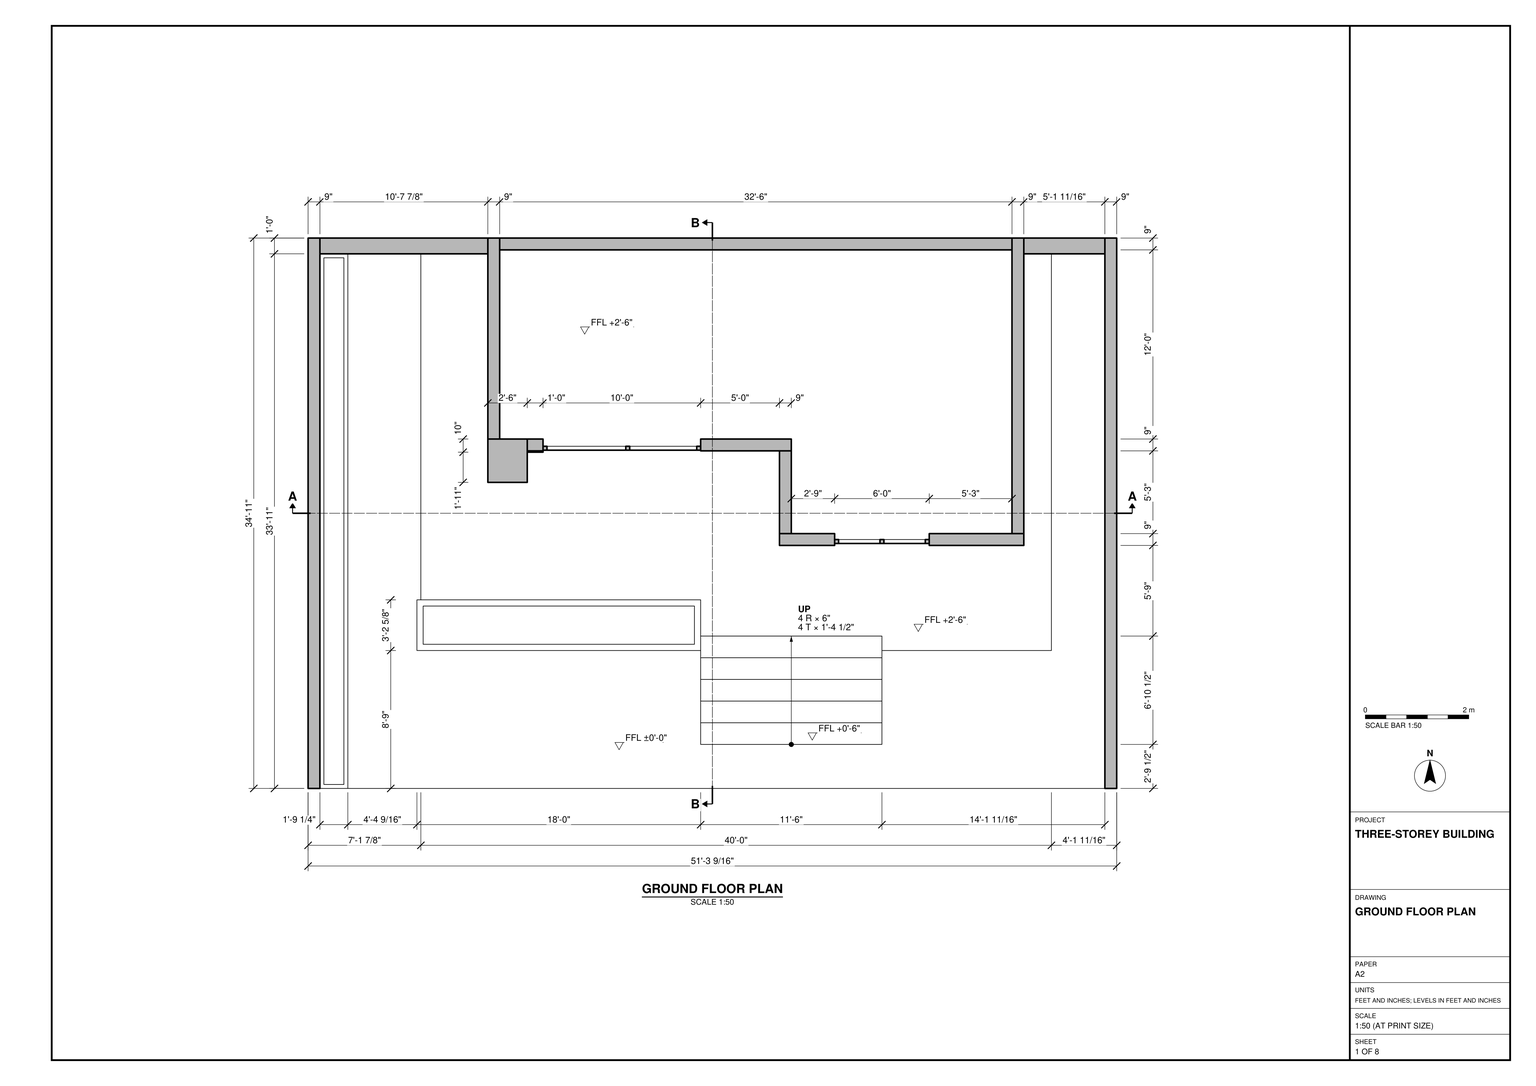
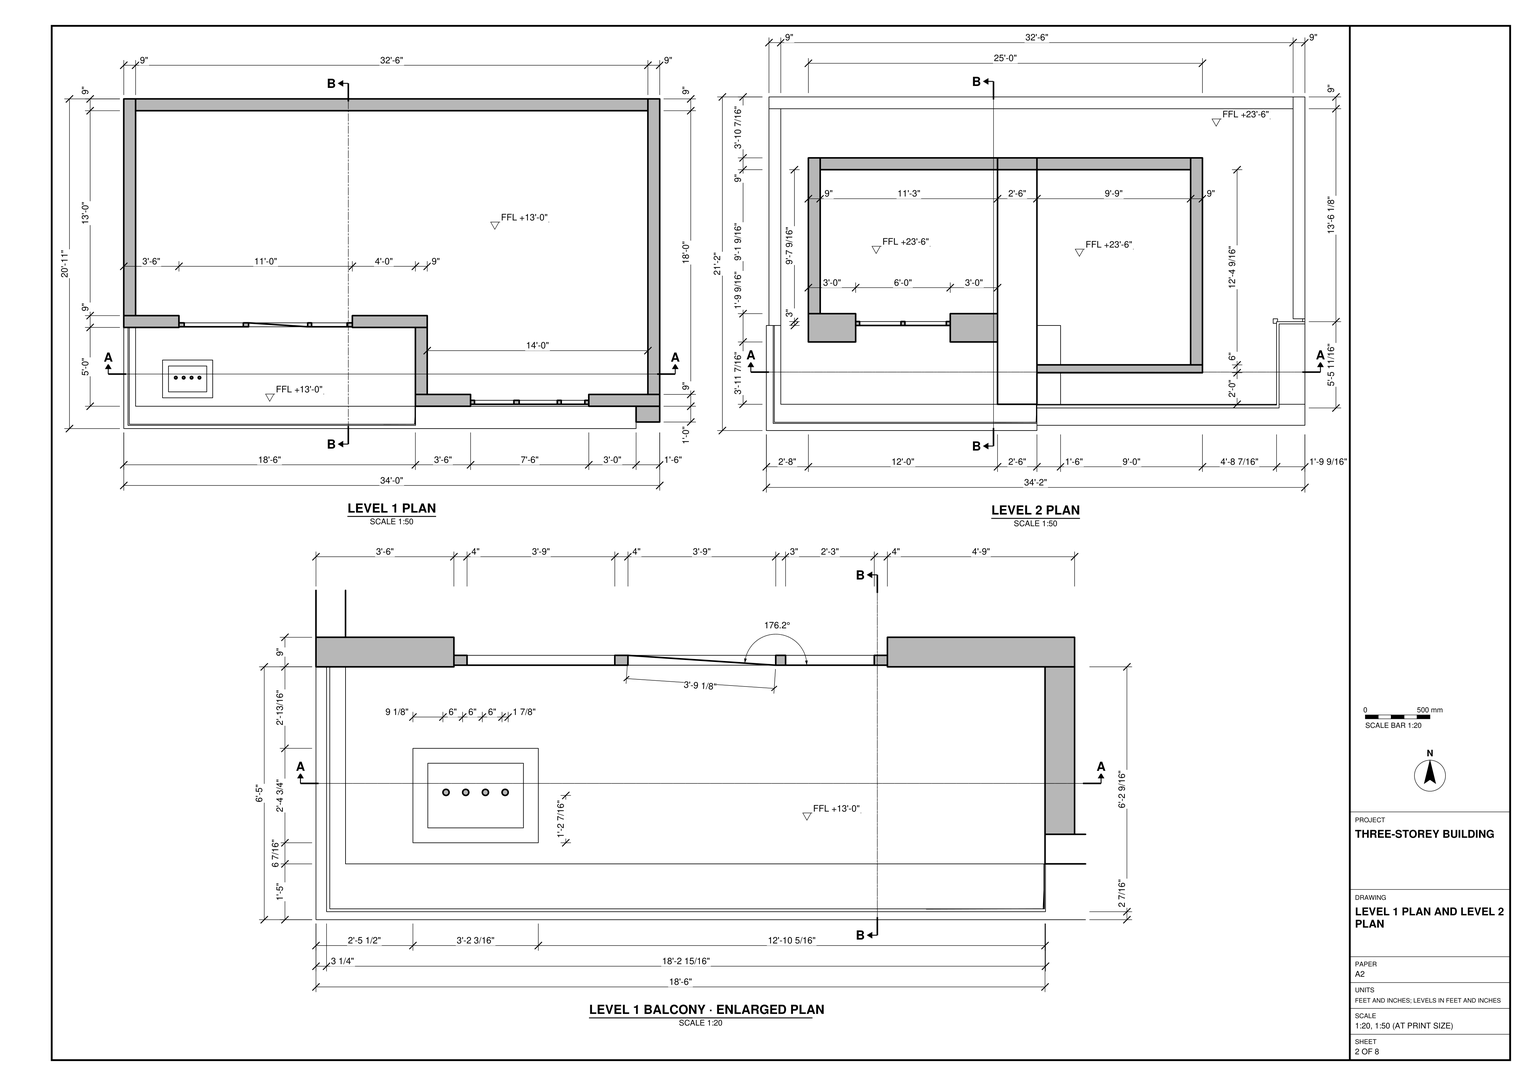
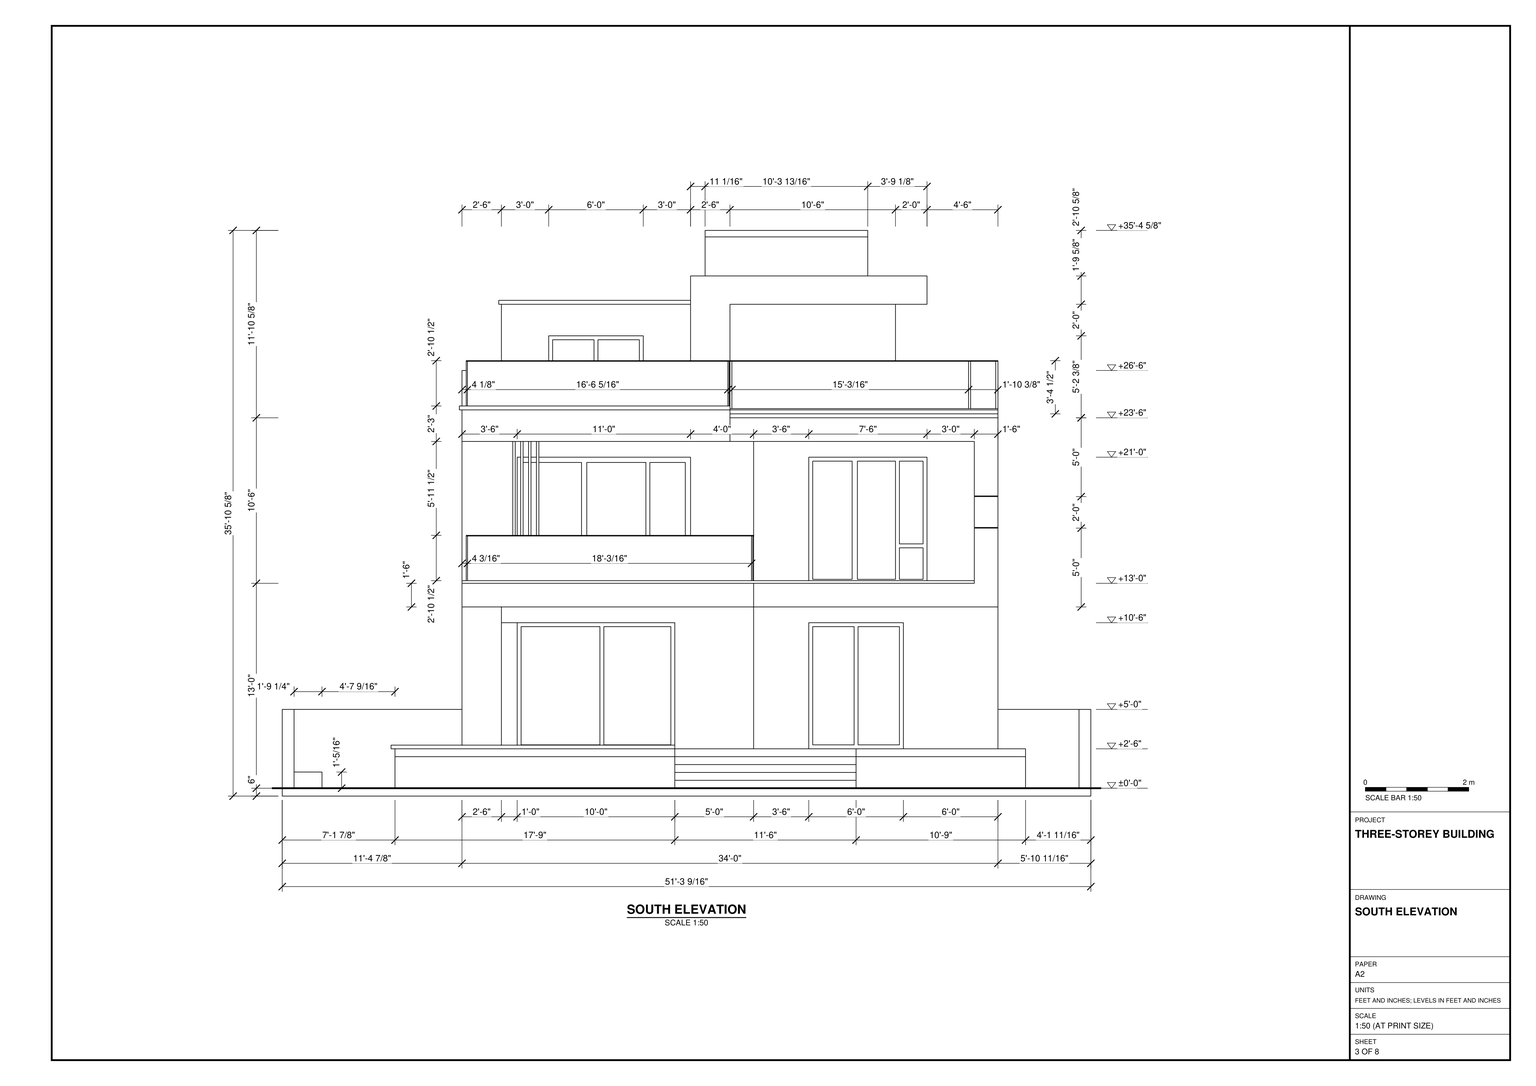
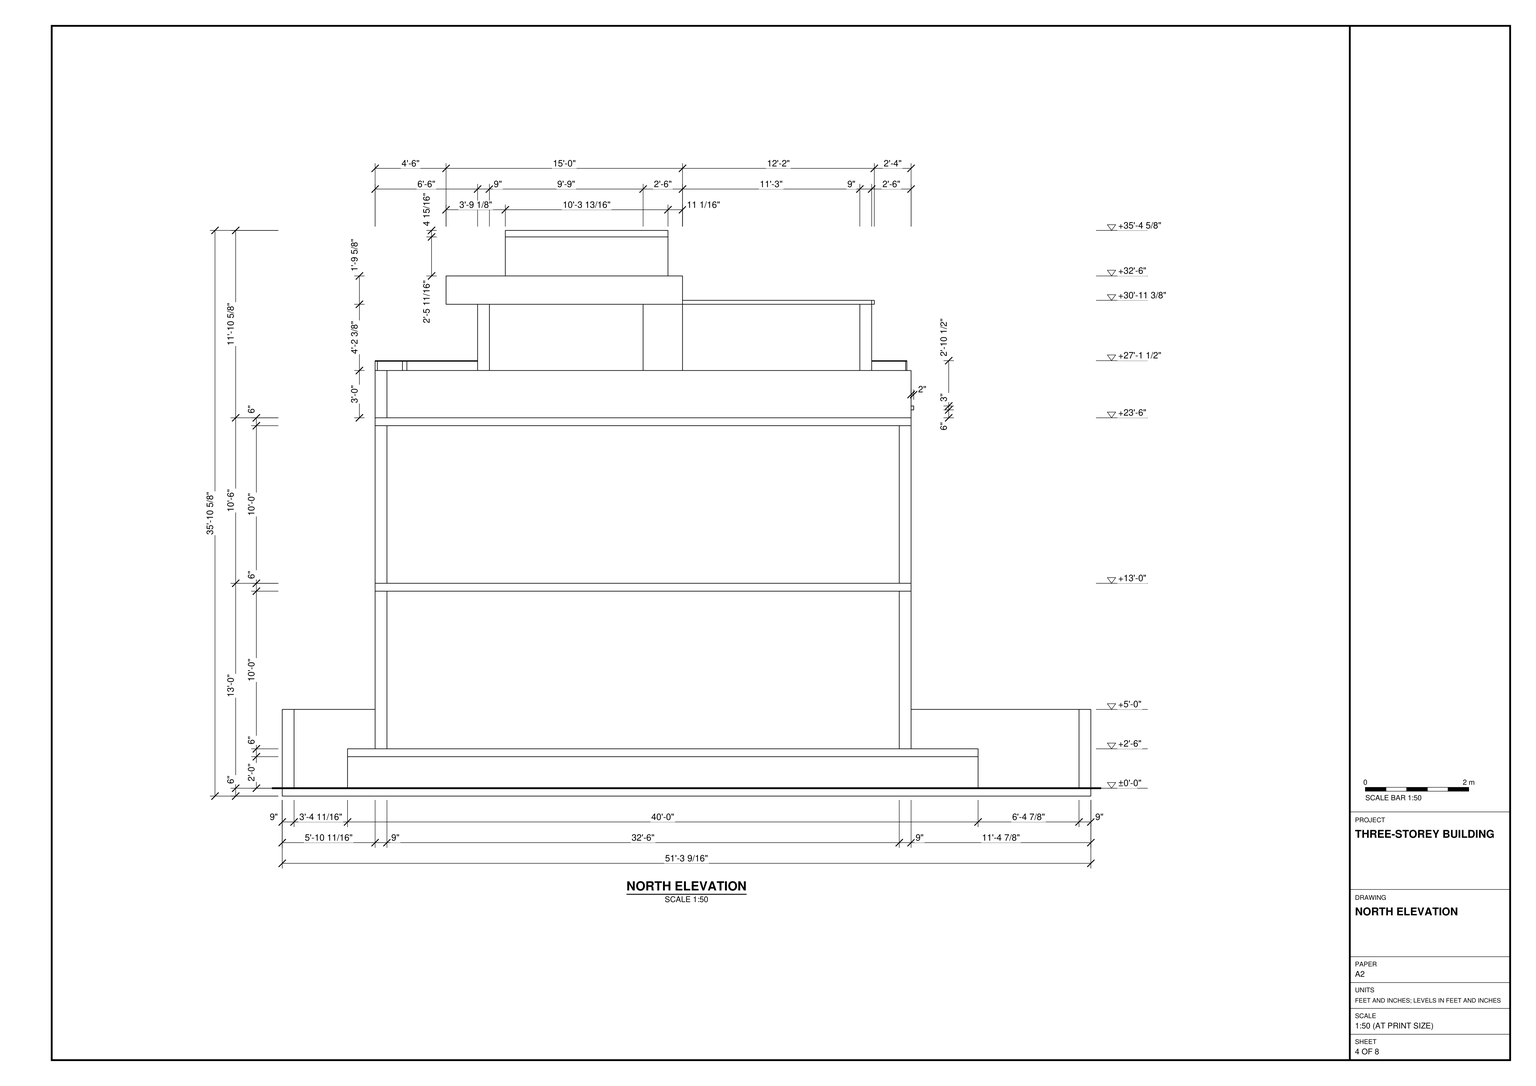
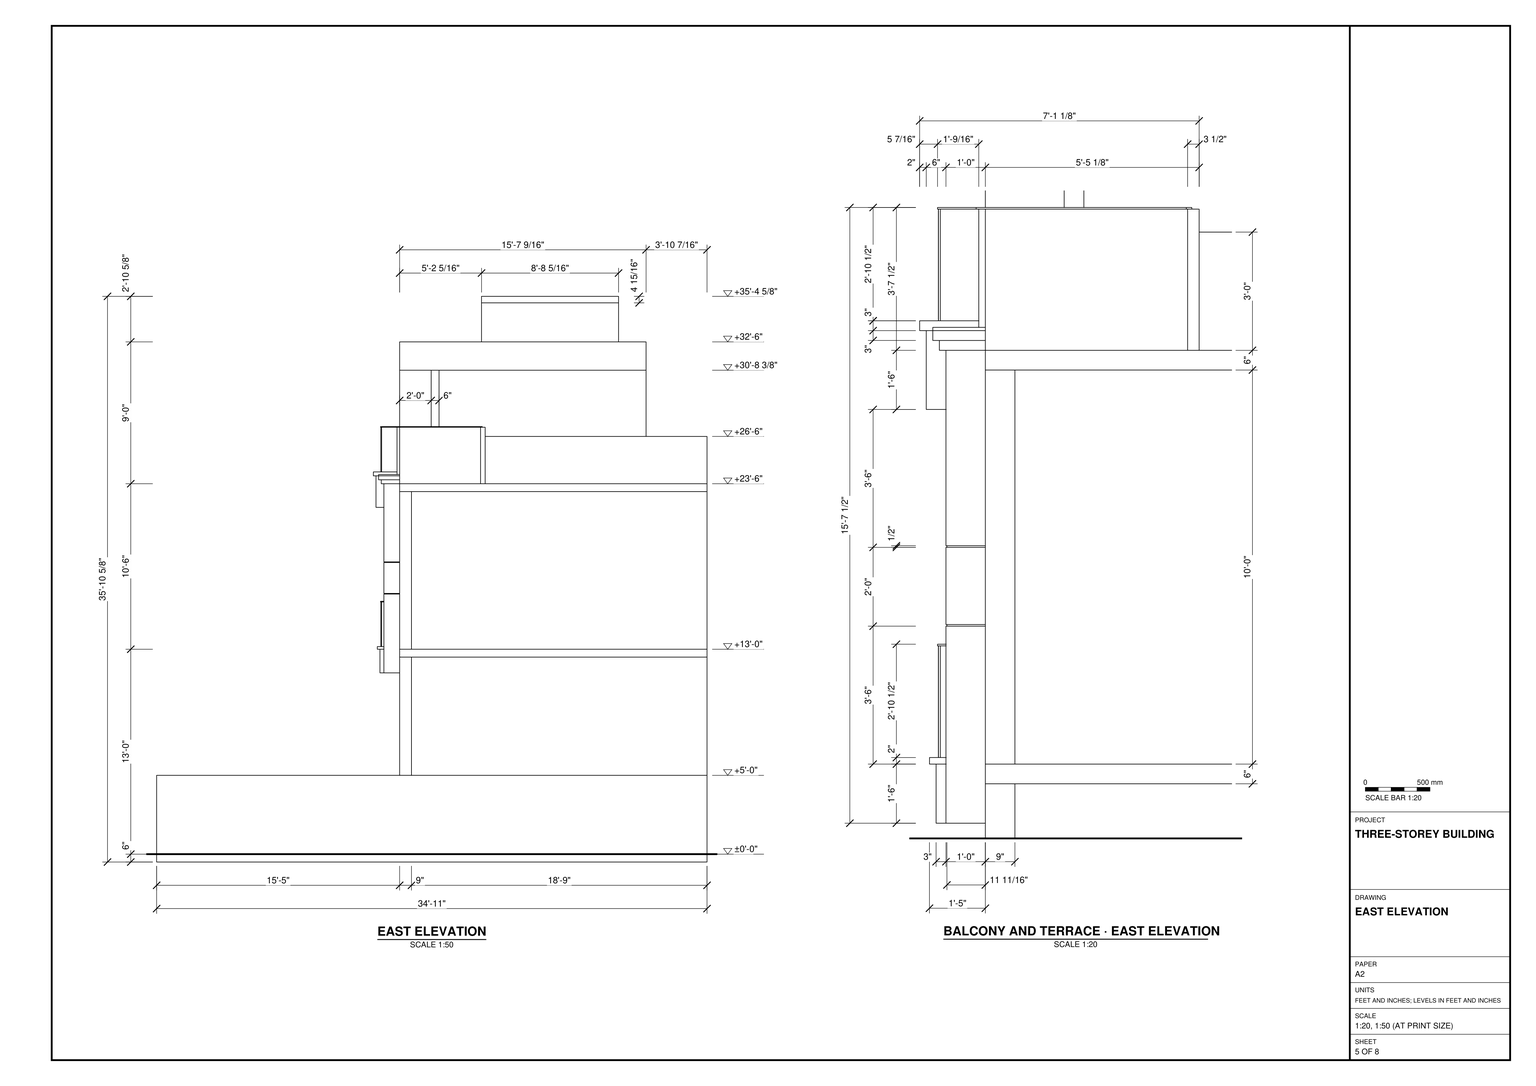
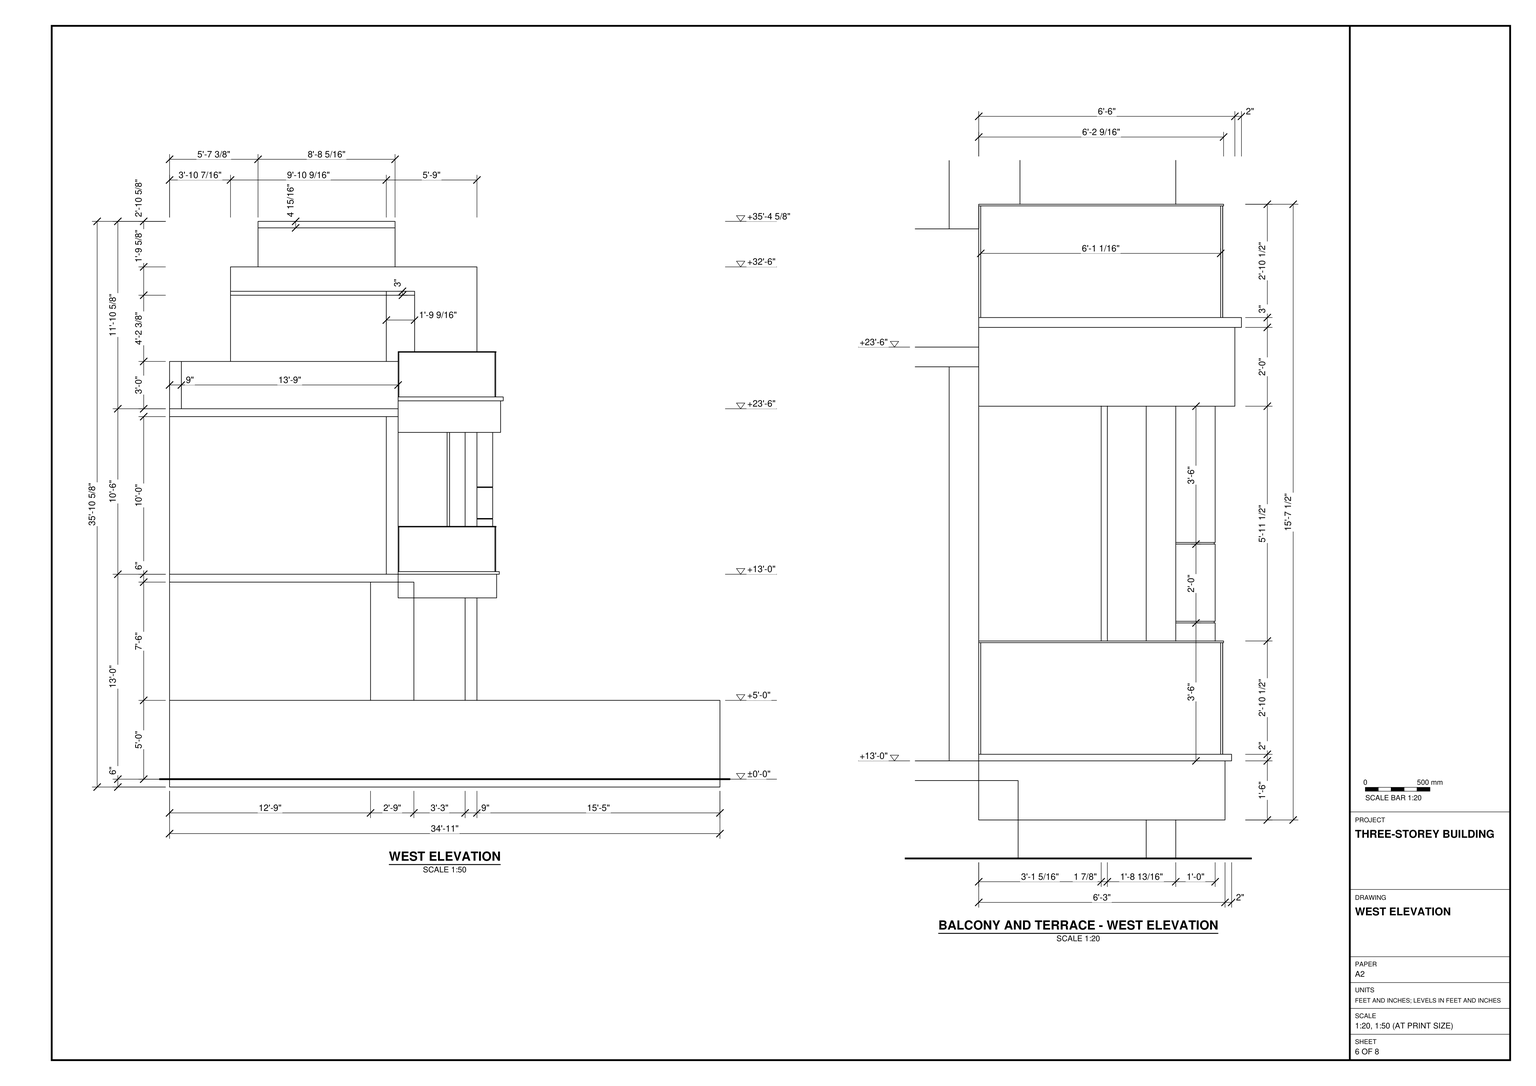
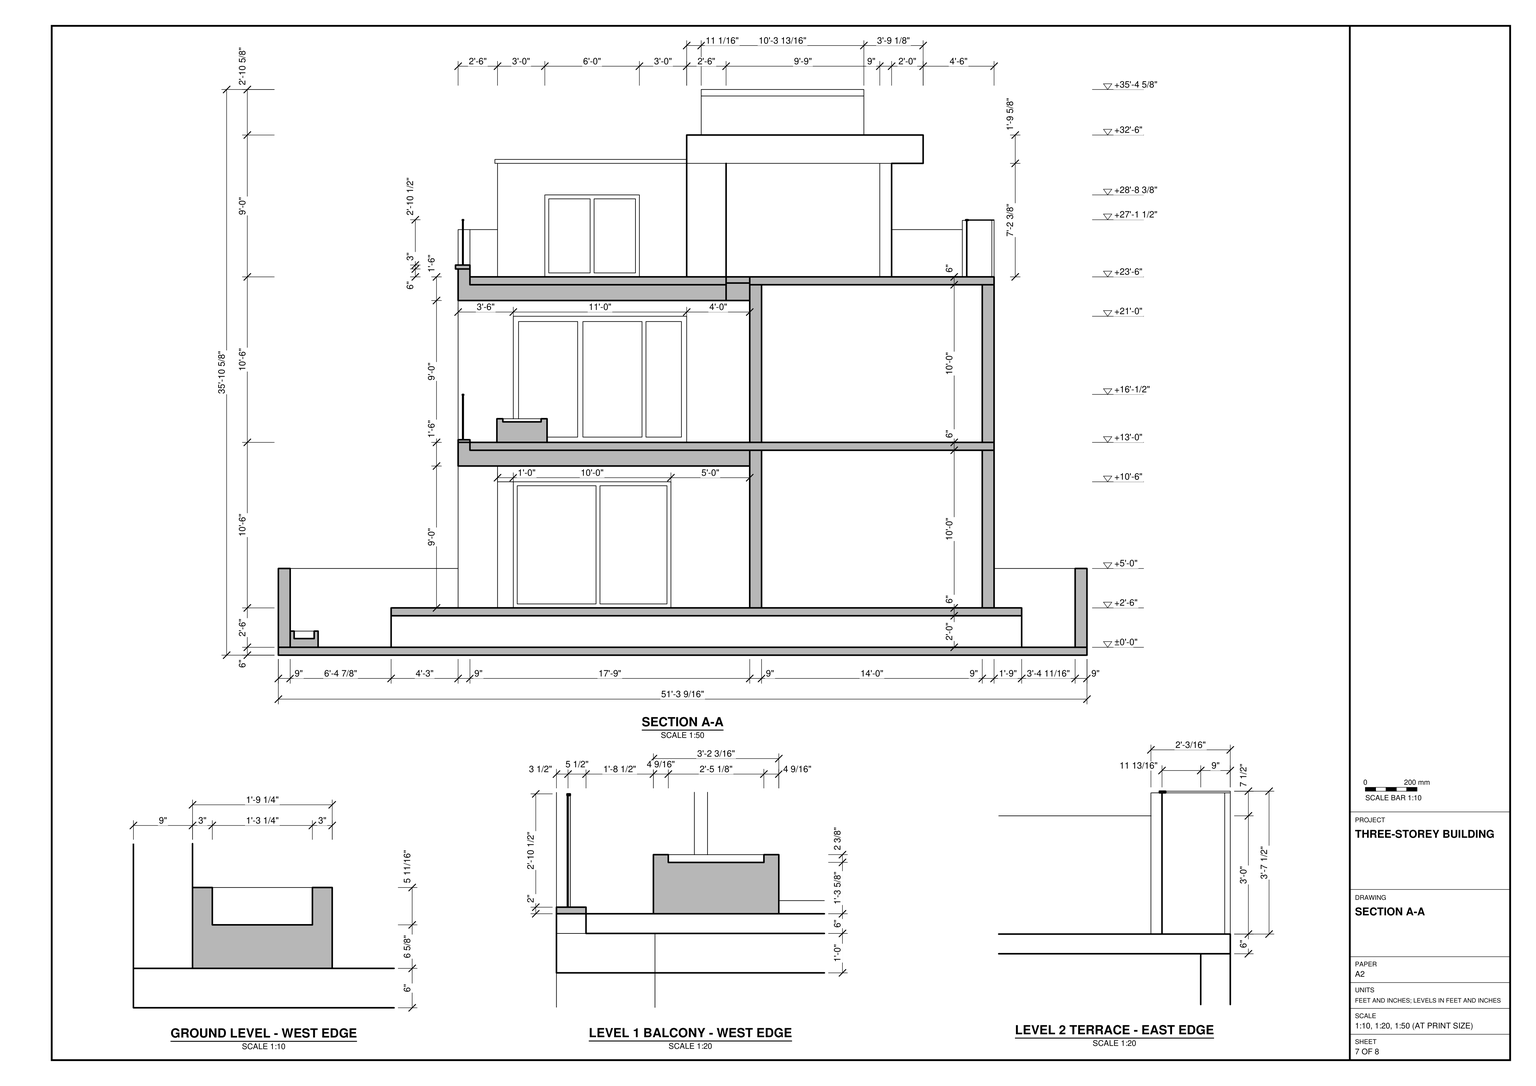
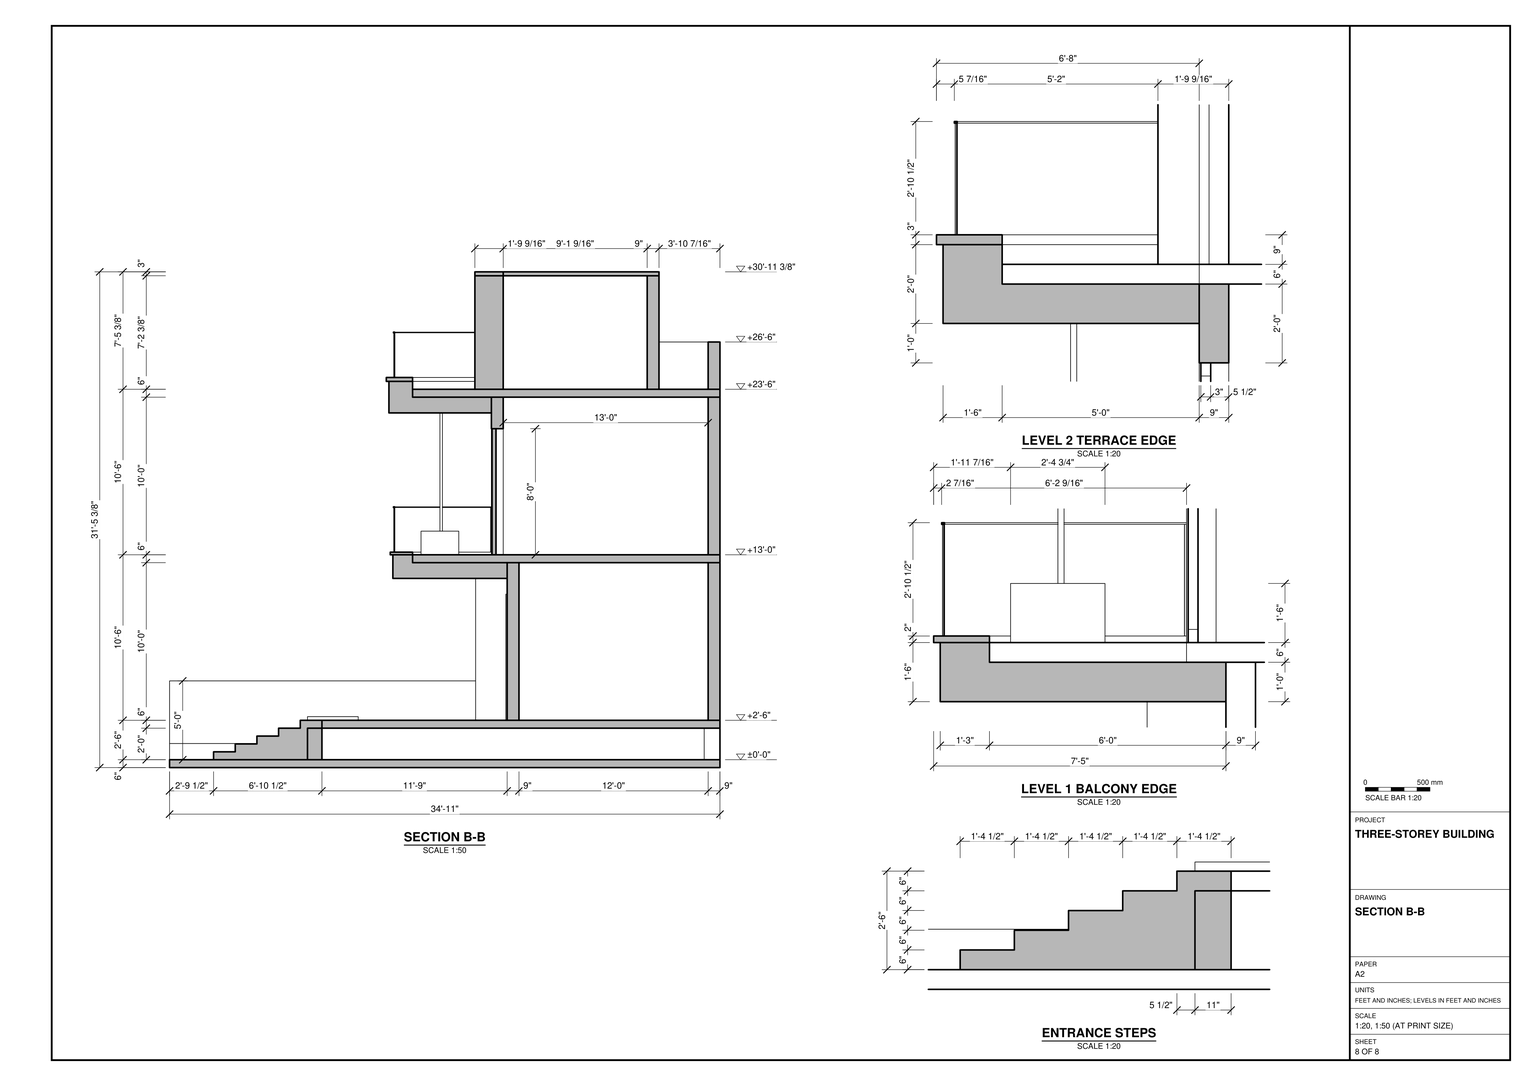
Build the three-storey building and its site in SketchUp from task_files/diagram_01.pdf. Work in feet and inches. Set the overall width to 51'-3 9/16", depth to 34'-11" and height, including the base slab, to 35'-10 5/8". Use the ground datum of ±0'-0" and the upper floor levels of +13'-0" and +23'-6".

Start with the site slab, the low boundary walls and the raised entrance platform at +2'-6". Leave the south approach open and place the broad flight of steps beside the long rectangular feature at the front of the platform. Follow the stepped wall line in plan: the west glazed bay sits farther back than the east bay. Use the wall thicknesses shown, including the 9" exterior walls, and model the frames and divisions within the glazed openings.

Build the floor slabs, the first-floor balcony across the recessed bay, and the set-back top floor with its larger terrace. Match the guards and their returns in plan. Use the south elevation to shape the roof, including the change in height and the projecting horizontal canopy. Include built-in joinery and main furniture where indicated. Decor and loose items may be any suitable library components. Keep walls, slabs, roof elements and each furniture or joinery piece in separate groups or components, and use components for repeated parts. Save one SketchUp model as output_files/three_storey_building_with_stepped_frontage.skp.

# SketchUp Ruby script. Lengths in inches.
U = 1.inch
M = Sketchup.active_model
def pt(a) = Geom::Point3d.new(a.map { |v| v * U })
def face(e, loops, mat)
  f = e.add_face(loops[0].map { |a| pt(a) })
  loops[1..].each { |l| e.add_face(l.map { |a| pt(a) }).erase! }
  f.material = f.back_material = mat if mat
  f
end
# faces: each face lists its corners as indices into pts; further lists are holes
def faces(e, pts, list, mat = nil) = list.each { |f| face(e, (f[0].is_a?(Array) ? f : [f]).map { |l| l.map { |i| pts[i] } }, mat) }
# xy, xz, yz: faces in a plane at the given z, y or x. An outline is a flat list of corners, or four numbers for a rectangle; further outlines are holes
def ring(l) = l.size == 4 ? [[l[0], l[1]], [l[2], l[1]], [l[2], l[3]], [l[0], l[3]]] : l.each_slice(2).to_a
def flat(e, list, mat, &to3) = list.each { |f| face(e, (f[0].is_a?(Array) ? f : [f]).map { |l| ring(l).map { |u, v| to3.(u, v) } }, mat) }
def xy(e, z, list, mat = nil) = flat(e, list, mat) { |x, y| [x, y, z] }
def xz(e, y, list, mat = nil) = flat(e, list, mat) { |x, z| [x, y, z] }
def yz(e, x, list, mat = nil) = flat(e, list, mat) { |y, z| [x, y, z] }
def lines(e, pts, list) = list.each { |a, b| e.add_line(pt(pts[a]), pt(pts[b])) }
# prism: a flat outline (further loops are holes) pulled along v
def prism(e, loops, v, mat = nil)
  f = face(e, loops, mat); d = Geom::Vector3d.new(v.map { |x| x * U })
  f.pushpull(f.normal.samedirection?(d) ? d.length : -d.length)
end
def box(e, o, s, mat = nil) = prism(e, [[o, [o[0] + s[0], o[1], o[2]], [o[0] + s[0], o[1] + s[1], o[2]], [o[0], o[1] + s[1], o[2]]]], [0, 0, s[2]], mat)
def at(x, y, z, deg = 0) = Geom::Transformation.translation(pt([x, y, z])) * Geom::Transformation.rotation(ORIGIN, Z_AXIS, deg.degrees)
def axes(o, x, y, z) = Geom::Transformation.new([*x, 0, *y, 0, *z, 0, *pt(o).to_a, 1])
def part(name) = M.definitions.add(name)
# library, detail: a bought-in or finely detailed component or shape, given as its bounding box
def library(name, o, s) = part(name).tap { |d| box(d.entities, o, s) }
def detail(e, o, s) = box(e.add_group.entities, o, s)
def put(e, d, t, mat = nil) = e.add_instance(d, t).tap { |i| i.material = mat if mat }
def group(e, t, mat = nil) = e.add_group.tap { |g| g.transformation = t; g.material = mat if mat }.entities
root = M.entities
M.materials.add("[Color D01]").color = [234, 222, 187]
M.materials.add("[Color D06]").color = [193, 144, 0]
M.materials.add("[Color E01]").color = [255, 255, 204]
M.materials.add("[Color M09]").color = [0, 0, 0]
M.materials.add("[Grass Dark Green]").color = [106, 157, 55]
M.materials.add("[Pavers Modular Brick]").color = [175, 152, 152]
M.materials.add("[Polished Concrete New]").color = [200, 200, 203]
M.materials.add("[Stone Brushed Khaki]").color = [196, 171, 115]
M.materials.add("[Translucent Glass Gold]").color = [254, 241, 255]
M.materials["[Translucent Glass Gold]"].alpha = 0.6
M.materials.add("[Translucent Glass Gray]").color = [128, 128, 128]
M.materials["[Translucent Glass Gray]"].alpha = 0.5
c1 = part("Group\#38")
prism(c1.entities,[[[1.02,0.61,0],[1,0,0],[0,0.04,0],[0.02,0.64,0]]],[0,0,34])
c2 = part("Group\#41")
xy(c2.entities,0,[[0,0,0,74.5625,0.98,74.5625,0.98,0.87,218.4375,0.87,218.4375,14.5625,218.92,14.5625,218.92,0]])
xy(c2.entities,0.5,[[0,0,218.92,0,218.92,14.5625,218.61,14.5625,218.61,0.87,0.98,0.87,0.98,74.5625,0,74.5625]])
xz(c2.entities,0,[[0,0,218.92,0.5]])
xz(c2.entities,0.87,[[0.98,0,217.07,0.5],[217.07,0,217.07,0.5,218.61,0.5,218.4375,0]])
xz(c2.entities,14.5625,[[218.4375,0,218.61,0.5,218.92,0.5,218.92,0]])
xz(c2.entities,74.5625,[[0,0,0.98,0.5]])
yz(c2.entities,0,[[0,0,74.5625,0.5]])
yz(c2.entities,0.98,[[0.87,0,74.5625,0.5]])
yz(c2.entities,218.92,[[0,0,14.5625,0.5]])
p = [[218.4375,0.87,0],[218.61,0.87,0.5],[218.61,14.5625,0.5],[218.4375,14.5625,0]]
faces(c2.entities,p,[[0,1,2,3]])
c3 = part("Group\#56")
box(c3.entities,[0,0,0],[1.59,2,40])
c4 = part("Group\#72")
prism(c4.entities,[[[1.41,1.75,0],[1.6,1.6,0],[1.75,1.41,0],[1.84,1.18,0],[1.875,0.9375,0],[1.84,0.69,0],[1.75,0.47,0],[1.6,0.27,0],[1.41,0.125,0],[1.18,0.03,0],[0.9375,0,0],[0.69,0.03,0],[0.47,0.125,0],[0.27,0.27,0],[0.125,0.47,0],[0.03,0.69,0],[0,0.9375,0],[0.03,1.18,0],[0.125,1.41,0],[0.27,1.6,0],[0.47,1.75,0],[0.69,1.84,0],[0.9375,1.875,0],[1.18,1.84,0]]],[0,0,97.3125])
xy(root,294,[[340.85,169,544.85,185]])
xy(root,295,[[340.85,169,544.85,185]],"[Color M09]")
xz(root,169,[[340.85,294,544.85,295]],"[Color M09]")
xz(root,185,[[340.85,294,544.85,295]])
yz(root,340.85,[[169,294,185,295]])
yz(root,544.85,[[169,294,185,295]])
g1 = group(root,at(85.85,176,6),"[Color D06]")
box(g1,[0,-71,0],[480,314,24])
g2 = group(root,at(85.85,116,30),"[Stone Brushed Khaki]")
prism(g2,[[[0,-11,0],[0,303,0],[480,303,0],[480,-11,0],[351,-11,0],[351,0,0],[213,0,0],[213,-11,0]]],[0,0,6])
g3 = group(root,at(358.85,185,36),"[Color D01]")
prism(g3,[[[42,9,0],[0,9,0],[0,9,120],[186,9,120],[186,9,0],[114,9,0],[114,9,96],[42,9,96]]],[0,-9,0])
g4 = group(root,at(535.85,194,36),"[Color D01]")
box(g4,[0,0,0],[9,225,120])
g5 = group(root,at(358.85,194,36),"[Color D01]")
box(g5,[0,0,0],[9,63,120])
g6 = group(root,at(400.85,186.5,36),"[Color M09]")
prism(g6,[[[72,3,0],[0,3,0],[0,3,96],[72,3,96]],[[34.5,3,3],[34.5,3,93],[3,3,93],[3,3,3]],[[69,3,93],[37.5,3,93],[37.5,3,3],[69,3,3]]],[0,-3,0])
g7 = group(root,at(438.35,186.5,39),"[Translucent Glass Gray]")
xz(g7,0,[[0,0,31.5,90]])
g8 = group(root,at(403.85,186.5,39),"[Translucent Glass Gray]")
xz(g8,0,[[0,0,31.5,90]])
g9 = group(root,at(154.85,257,36),"[Color D06]")
prism(g9,[[[12,0,0],[24,0,0],[24,0,96],[144,0,96],[144,0,0],[213,0,0],[213,0,120],[12,0,120]]],[0,9,0])
g10 = group(root,at(178.85,257.5,36),"[Color M09]")
prism(g10,[[[0,3,0],[0,3,96],[120,3,96],[120,3,0]],[[63,3,3],[63,3,93],[3,3,93],[3,3,3]],[[117,3,93],[66,3,93],[66,3,3],[117,3,3]]],[0,-3,0])
g11 = group(root,at(244.85,257.5,39),"[Translucent Glass Gray]")
xz(g11,0,[[0,0,51,90]])
g12 = group(root,at(181.85,257.5,39),"[Translucent Glass Gray]")
xz(g12,0,[[0,0,60,90]])
g13 = group(root,at(136.85,245,36),"[Color D01]")
box(g13,[0,-12,0],[30,33,120])
g14 = group(root,at(166.85,256,36),"[Color D01]")
box(g14,[0,0,0],[12,1,96])
g15 = group(root,at(136.85,266,36),"[Color E01]")
box(g15,[0,0,0],[9,153,120])
g16 = group(root,at(136.85,185,144),"[Color D01]")
xy(g16,0,[[0,-15,0,60,30,60,30,72,222,72,222,-15]])
xy(g16,12,[[9,0,222,0,222,72,30,72,30,60,9,60]])
xy(g16,18,[[0,-15,222,-15,222,0,9,0,9,60,0,60]])
xz(g16,-15,[[0,0,222,18]])
xz(g16,0,[[9,12,222,18]])
xz(g16,60,[[0,0,30,12],[0,12,9,18]])
xz(g16,72,[[30,0,222,12]])
yz(g16,0,[[-15,0,60,18]])
yz(g16,9,[[0,12,60,18]])
yz(g16,30,[[60,0,72,12]])
yz(g16,222,[[-15,0,72,0,72,12,0,12,0,18,-15,18]])
g17 = group(root,at(136.85,185,156),"[Color D01]")
prism(g17,[[[408,234,0],[408,0,0],[9,0,0],[9,60,0],[0,60,0],[0,234,0]]],[0,0,6])
g18 = group(root,at(358.85,185,162),"[Color D01]")
prism(g18,[[[42,9,0],[0,9,0],[0,9,120],[186,9,120],[186,9,0],[132,9,0],[132,9,96],[42,9,96]]],[0,-9,0])
g19 = group(root,at(400.85,186.5,162),"[Color M09]")
prism(g19,[[[0,3,0],[0,3,96],[90,3,96],[90,3,0]],[[3,3,3],[33,3,3],[33,3,93],[3,3,93]],[[37,3,93],[37,3,3],[66,3,3],[66,3,93]],[[87,3,93],[69,3,93],[69,3,30],[87,3,30]],[[87,3,3],[87,3,27],[69,3,27],[69,3,3]]],[0,-3,0])
g20 = group(root,at(469.85,186.5,192),"[Translucent Glass Gray]")
xz(g20,0,[[0,0,18,63]])
g21 = group(root,at(469.85,186.5,165),"[Translucent Glass Gray]")
xz(g21,0,[[0,0,18,24]])
g22 = group(root,at(437.85,186.5,165),"[Translucent Glass Gray]")
xz(g22,0,[[0,0,29,90]])
g23 = group(root,at(403.85,186.5,165),"[Translucent Glass Gray]")
xz(g23,0,[[0,0,30,90]])
g24 = group(root,at(358.85,194,162),"[Color D01]")
box(g24,[0,0,0],[9,51,120])
g25 = group(root,at(136.85,245,162),"[Color D01]")
prism(g25,[[[0,0,0],[42,0,0],[42,0,96],[174,0,96],[174,0,0],[231,0,0],[231,0,120],[0,0,120]]],[0,9,0])
g26 = group(root,at(178.85,245.5,162),"[Color M09]")
prism(g26,[[[0,3,96],[132,3,96],[132,3,0],[0,3,0]],[[49,3,4],[49,3,92],[4,3,92],[4,3,4]],[[98,3,92],[53,3,92],[53,3,4],[98,3,4]],[[128,3,92],[101,3,92],[101,3,4],[128,3,4]]],[0,-3,0])
g27 = group(root,at(279.85,245.5,166),"[Translucent Glass Gray]")
xz(g27,0,[[0,0,27,88]])
g28 = group(root,at(231.85,245.5,166),"[Translucent Glass Gray]")
p = [[0,3,88],[45,0,88],[45,0,0],[0,3,0]]
faces(g28,p,[[0,1,2,3]])
g29 = group(root,at(182.85,245.5,166),"[Translucent Glass Gray]")
xz(g29,0,[[0,0,45,88]])
g30 = group(root,at(535.85,194,162),"[Color D01]")
box(g30,[0,0,0],[9,225,120])
g31 = group(root,at(136.85,254,162),"[Color D01]")
box(g31,[0,0,0],[9,165,120])
g32 = group(root,at(136.85,185,282),"[Color D01]")
xy(g32,0,[[9,0,9,60,0,60,0,234,408,234,408,0,222,0,222,60,204,60,204,0]])
xy(g32,1.3125,[[204,0,222,60]])
xy(g32,6,[[9,0,408,0,408,234,0,234,0,60,9,60]])
xz(g32,0,[[9,0,204,6],[222,0,408,6],[204,1.3125,222,6]])
xz(g32,60,[[0,0,9,6],[204,0,222,1.3125]])
xz(g32,234,[[0,0,408,6]])
yz(g32,0,[[60,0,234,6]])
yz(g32,9,[[0,0,60,6]])
yz(g32,204,[[0,0,60,1.3125]])
yz(g32,222,[[0,0,60,1.3125]])
yz(g32,408,[[0,0,234,6]])
g33 = group(root,at(358.85,173,144),"[Color D06]")
xy(g33,0,[[0,0,186,12]])
xy(g33,18,[[0,0,168,12]])
xy(g33,60,[[168,0,186,0.3],[168,0.3,168.3,12],[168.3,0.3,185.7,12],[185.7,0.3,186,12]])
xy(g33,60.5,[[168,0,186,0.3],[168,0.3,168.3,12],[168.3,0.3,185.7,12],[185.7,0.3,186,12]])
xy(g33,84,[[168,0,186,0.3],[168,0.3,168.3,12],[168.3,0.3,185.7,12],[185.7,0.3,186,12]])
xy(g33,84.5,[[168,0,186,0.3],[168,0.3,168.3,12],[168.3,0.3,185.7,12],[185.7,0.3,186,12]])
xy(g33,126,[[-18,0,-18,72,0,72,0,12,168,12,168,0]])
xy(g33,144,[[-18,0,186,0,186,12,0,12,0,72,-18,72]])
xz(g33,0,[[0,0,186,0,186,60,168,60,168,18,0,18],[168,60.5,186,84],[168,84.5,186,84.5,186,144,-18,144,-18,126,168,126]])
xz(g33,0.3,[[168.3,60,185.7,60.5],[168.3,84,185.7,84.5]])
xz(g33,12,[[0,0,0,18,168,18,168,60,186,60,186,0],[168.3,60,185.7,60.5],[168,60.5,186,84],[168.3,84,185.7,84.5],[168,84.5,168,126,0,126,0,144,186,144,186,84.5]])
xz(g33,72,[[-18,126,0,144]])
yz(g33,-18,[[0,126,72,144]])
yz(g33,0,[[0,0,12,18],[12,126,72,144]])
yz(g33,168,[[0,18,12,60],[0,60.5,12,84],[0,84.5,12,126]])
yz(g33,168.3,[[0.3,60,12,60.5],[0.3,84,12,84.5]])
yz(g33,185.7,[[0.3,60,12,60.5],[0.3,84,12,84.5]])
yz(g33,186,[[0,0,12,60],[0,60.5,12,84],[0,84.5,12,144]])
g34 = group(root,at(136.85,173,270),"[Color D01]")
xy(g34,0,[[0,-6,204,72]])
xy(g34,12,[[9,12,204,72]])
xy(g34,24,[[0,-6,204,-6,204,12,9,12,9,72,0,72]])
xz(g34,-6,[[0,0,204,24]])
xz(g34,12,[[9,12,204,24]])
xz(g34,72,[[0,0,204,12],[0,12,9,24]])
yz(g34,0,[[-6,0,72,24]])
yz(g34,9,[[12,12,72,24]])
yz(g34,204,[[-6,0,72,0,72,12,12,12,12,24,-6,24]])
g35 = group(root,at(136.85,168,162),"[Color D06]")
prism(g35,[[[0,0,0],[0,77,0],[9,77,0],[9,17,0],[390,17,0],[390,0,0]]],[0,0,2])
g36 = group(root,at(358.26,171.3,164),"[Translucent Glass Gold]")
p = [[0,0,34],[0.59,13.7,34],[0.59,13.7,0],[0,0,0]]
faces(g36,p,[[0,1,2,3]],"[Translucent Glass Gray]")
put(root,c1,at(357.24,170.6875,164),"[Color M09]")
put(root,c1,at(140.05,170.6875,164),"[Color M09]")
g37 = group(root,at(141.05,170.6875,164),"[Translucent Glass Gold]")
p = [[0,0,0],[0,0,34],[216.21,0.64,34],[216.21,0.64,0]]
faces(g37,p,[[0,1,2,3]],"[Translucent Glass Gray]")
put(root,c1,at(140.05,244.36,164),"[Color M09]")
g38 = group(root,at(140.36,171.32,164),"[Translucent Glass Gold]")
p = [[0,73.0625,34],[0.02,0,34],[0.02,0,0],[0,73.0625,0]]
faces(g38,p,[[0,1,2,3]],"[Translucent Glass Gray]")
put(root,c2,at(140.07,170.4375,198),"[Color M09]")
g39 = group(root,at(340.85,171,288),"[Color D06]")
box(g39,[0,0,0],[204,14,3])
g40 = group(root,at(134.85,165,294),"[Color D06]")
prism(g40,[[[0,0,0],[0,80,0],[11,80,0],[11,20,0],[206,20,0],[206,0,0]]],[0,0,3])
g41 = group(root,at(140.05,170.4375,297),"[Translucent Glass Gray]")
g42 = group(g41,at(0.92,0.25,0),"[Translucent Glass Gold]")
p = [[0,0,0],[0,0,34],[198.3,0.64,34],[198.3,0.64,0]]
faces(g42,p,[[0,1,2,3]],"[Translucent Glass Gray]")
g43 = group(g41,at(0.29,0.88,0),"[Translucent Glass Gold]")
p = [[0,73.0625,34],[0.02,0,34],[0.02,0,0],[0,73.0625,0]]
faces(g43,p,[[0,1,2,3]],"[Translucent Glass Gray]")
g44 = group(g41,at(200.13,0.86,0),"[Translucent Glass Gold]")
p = [[0,0,34],[0.54,13.7,34],[0.54,13.7,0],[0,0,0]]
faces(g44,p,[[0,1,2,3]],"[Translucent Glass Gray]")
put(g41,c1,axes([199.19,0.25,0],[0.91714,0,0],[0,1,0],[0,0,1]),"[Color M09]")
put(g41,c1,axes([0,0.25,0],[0.91714,0,0],[0,1,0],[0,0,1]),"[Color M09]")
put(g41,c2,axes([0.02,0,34],[0.91714,0,0],[0,1,0],[0,0,1]),"[Color M09]")
put(g41,c1,axes([0,73.92,0],[0.91714,0,0],[0,1,0],[0,0,1]),"[Color M09]")
g45 = group(root,at(310.85,185,288),"[Color D01]")
xy(g45,0,[[0,0,30,187.59],[30,24,156,30],[147,30,156,187.59]])
xy(g45,86.4,[[30,0,30,24,156,24,156,187.59,180,187.59,180,0],[30,30,147,187.59],[147,30,156,187.59]])
xy(g45,108,[[0,0,180,187.59]])
xz(g45,0,[[0,0,30,0,30,86.4,180,86.4,180,108,0,108]])
xz(g45,24,[[30,0,156,86.4]])
xz(g45,30,[[30,0,147,86.4],[147,0,156,86.4]])
xz(g45,187.59,[[0,0,0,108,180,108,180,86.4,30,86.4,30,0],[147,0,156,86.4]])
yz(g45,0,[[0,0,187.59,108]])
yz(g45,30,[[0,0,24,86.4],[24,0,30,86.4],[30,0,187.59,86.4]])
yz(g45,147,[[30,0,187.59,86.4]])
yz(g45,156,[[24,0,30,86.4],[30,0,187.59,86.4]])
yz(g45,180,[[0,86.4,187.59,108]])
g46 = group(root,at(166.85,245,288),"[Color D01]")
prism(g46,[[[0,-12.5625,0],[36,-12.5625,0],[36,-12.5625,62.4],[108,-12.5625,62.4],[108,-12.5625,0],[144,-12.5625,0],[144,-12.5625,86.4],[0,-12.5625,86.4]]],[0,21.5625,0])
g47 = group(root,at(202.85,245,288),"[Color M09]")
prism(g47,[[[0,3,0],[0,3,62.4],[72,3,62.4],[72,3,0]],[[34.5,3,3],[34.5,3,59.4],[3,3,59.4],[3,3,3]],[[69,3,59.4],[37.5,3,59.4],[37.5,3,3],[69,3,3]]],[0,-3,0])
g48 = group(root,at(240.35,245,291),"[Translucent Glass Gray]")
xz(g48,0,[[0,0,31.5,56.4]])
g49 = group(root,at(205.85,245,291),"[Translucent Glass Gray]")
xz(g49,0,[[0,0,31.5,56.4]])
g50 = group(root,at(164.85,243,374.4),"[Color D06]")
box(g50,[0,-10.5625,0],[146,21.5625,3])
g51 = group(root,at(166.85,254,288),"[Color D01]")
box(g51,[0,0,0],[9,118.59,86.4])
g52 = group(root,at(175.85,363.59,288),"[Color D01]")
box(g52,[0,0,0],[282,9,86.4])
g53 = group(root,at(166.85,254,374.4),"[Color D01]")
box(g53,[0,0,0],[144,118.59,3])
g54 = group(root,at(321.91,247.33,396),"[Color D06]")
xy(g54,0,[[0,0,123.8125,104.3125]])
xy(g54,29.7,[[0,0,123.8125,104.3125]])
xy(g54,34.65,[[0,0,123.8125,104.3125]])
xz(g54,0,[[0,0,123.8125,29.7],[0,29.7,123.8125,34.65]])
xz(g54,104.3125,[[0,0,123.8125,29.7],[0,29.7,123.8125,34.65]])
yz(g54,0,[[0,0,104.3125,29.7],[0,29.7,104.3125,34.65]])
yz(g54,123.8125,[[0,0,104.3125,29.7],[0,29.7,104.3125,34.65]])
put(root,c3,at(340.72,183,291),"[Color M09]")
put(root,c3,at(522.47,183,291),"[Color M09]")
g55 = group(root,at(342.3,183,291),"[Translucent Glass Gray]")
xz(g55,0,[[0,0,180.16,40]])
g56 = group(root,at(520.68,185,288))
xy(g56,0,[[0,61.59,3.375,65.1]])
xy(g56,43,[[0,61.59,3.375,65.1]],"[Color M09]")
xz(g56,61.59,[[0,0,3.375,43]],"[Color M09]")
xz(g56,65.1,[[0,0,3.375,43]],"[Color M09]")
yz(g56,0,[[61.59,0,65.1,43]],"[Color M09]")
yz(g56,3.375,[[61.59,0,65.1,43]],"[Color M09]")
yz(g56,3.375,[[0,0,61.59,43]],"[Translucent Glass Gray]")
g57 = group(root,at(535.85,250.1,288),"[Color D01]")
box(g57,[0,0,0],[9,168.9,36])
g58 = group(root,at(136.85,410,288),"[Color D01]")
box(g58,[0,0,0],[399,9,36])
g59 = group(root,at(136.85,245,288),"[Color D01]")
box(g59,[0,0,0],[9,165,36])
g60 = group(root,at(524.05,246.59,288))
xy(g60,0,[[19.1,0,20.79,3.5]])
xy(g60,43,[[19.1,0,20.79,3.5]],"[Color M09]")
xz(g60,0,[[19.1,0,20.79,43]],"[Color M09]")
xz(g60,0,[[0,0,19.1,43]],"[Translucent Glass Gray]")
xz(g60,3.5,[[19.1,0,20.79,43]],"[Color M09]")
yz(g60,19.1,[[0,0,3.5,43]],"[Color M09]")
yz(g60,20.79,[[0,0,3.5,43]],"[Color M09]")
g61 = group(root,at(340.85,169,291))
box(g61,[0,0,0],[204,16,3])
g62 = group(root,at(340.85,182.1875,331),"[Color M09]")
prism(g62,[[[184.33,63.99,0],[184.33,0,0],[0,0,0],[0,2.25,0],[182.41,2.25,0],[182.41,65.6875,0],[204,65.6875,0],[204,63.99,0]]],[0,0,0.5])
g63 = group(root,at(-73.125,-259.09,0),"[Pavers Modular Brick]")
box(g63,[73.125,259.09,0],[615.5625,419,6])
g64 = group(root,at(298.85,33.5,6),"[Polished Concrete New]")
prism(g64,[[[138,0,0],[138,82.5,0],[138,82.5,30],[138,66,30],[138,66,24],[138,49.5,24],[138,49.5,18],[138,33,18],[138,33,12],[138,16.5,12],[138,16.5,6],[138,0,6]]],[-138,0,0])
g65 = group(root,at(166.37,191.42,162),"[Color D01]")
xy(g65,0,[[0,0,38.1875,28.75]])
xy(g65,15.625,[[4.53,4.53,33.65,24.22]],"[Grass Dark Green]")
xy(g65,18,[[[0,0,38.1875,28.75],[4.53,4.53,33.65,24.22]]])
xz(g65,0,[[0,0,38.1875,18]])
xz(g65,4.53,[[4.53,15.625,33.65,18]])
xz(g65,24.22,[[4.53,15.625,33.65,18]])
xz(g65,28.75,[[0,0,38.1875,18]])
yz(g65,0,[[0,0,28.75,18]])
yz(g65,4.53,[[4.53,15.625,24.22,18]])
yz(g65,33.65,[[4.53,15.625,24.22,18]])
yz(g65,38.1875,[[0,0,28.75,18]])
g66 = group(root,at(82.85,105,36),"[Stone Brushed Khaki]")
xy(g66,0,[[0,0,216,38.6]])
xy(g66,1.26,[[4.74,4.74,211.26,33.86]],"[Grass Dark Green]")
xy(g66,2.79,[[[0,0,216,38.6],[4.74,4.74,211.26,33.86]]])
xz(g66,0,[[0,0,216,2.79]])
xz(g66,4.74,[[4.74,1.26,211.26,2.79]])
xz(g66,33.86,[[4.74,1.26,211.26,2.79]])
xz(g66,38.6,[[0,0,216,2.79]])
yz(g66,0,[[0,0,38.6,2.79]])
yz(g66,4.74,[[4.74,1.26,33.86,2.79]])
yz(g66,211.26,[[4.74,1.26,33.86,2.79]])
yz(g66,216,[[0,0,38.6,2.79]])
g67 = group(root,at(145.85,410,36),"[Color D01]")
box(g67,[0,0,0],[390,9,120])
g68 = group(root,at(145.85,410,162),"[Color D01]")
box(g68,[0,0,0],[390,9,120])
put(root,c4,at(193.5,205.84,177.625),"[Color M09]")
put(root,c4,at(187.5,205.84,177.625),"[Color M09]")
put(root,c4,at(181.5,205.84,177.625),"[Color M09]")
put(root,c4,at(175.5,205.84,177.625),"[Color M09]")
g69 = group(root,at(0,0,6))
box(g69,[0,0,0],[9,419,60])
g70 = group(root,at(606.5625,0,6))
box(g70,[0,0,0],[9,419,60])
g71 = group(root,at(565.85,407,6))
prism(g71,[[[0,0,0],[40.72,0,0],[40.72,0,60],[-21,0,60],[-21,0,30],[0,0,30]]],[0,12,0])
g72 = group(root,at(9,407,6))
prism(g72,[[[0,0,0],[76.85,0,0],[76.85,0,30],[127.85,0,30],[127.85,0,60],[0,0,60]]],[0,12,0])
g73 = group(root,at(9,0,6))
xy(g73,0,[[0,0,21.27,407]])
xy(g73,6.625,[[3.01,3.01,18.25,403.99]],"[Grass Dark Green]")
xy(g73,12.3125,[[[0,0,21.27,407],[3.01,3.01,18.25,403.99]]])
xz(g73,0,[[0,0,21.27,12.3125]])
xz(g73,3.01,[[3.01,6.625,18.25,12.3125]])
xz(g73,403.99,[[3.01,6.625,18.25,12.3125]])
xz(g73,407,[[0,0,21.27,12.3125]])
yz(g73,0,[[0,0,407,12.3125]])
yz(g73,3.01,[[3.01,6.625,403.99,12.3125]])
yz(g73,18.25,[[3.01,6.625,403.99,12.3125]])
yz(g73,21.27,[[0,0,407,12.3125]])
